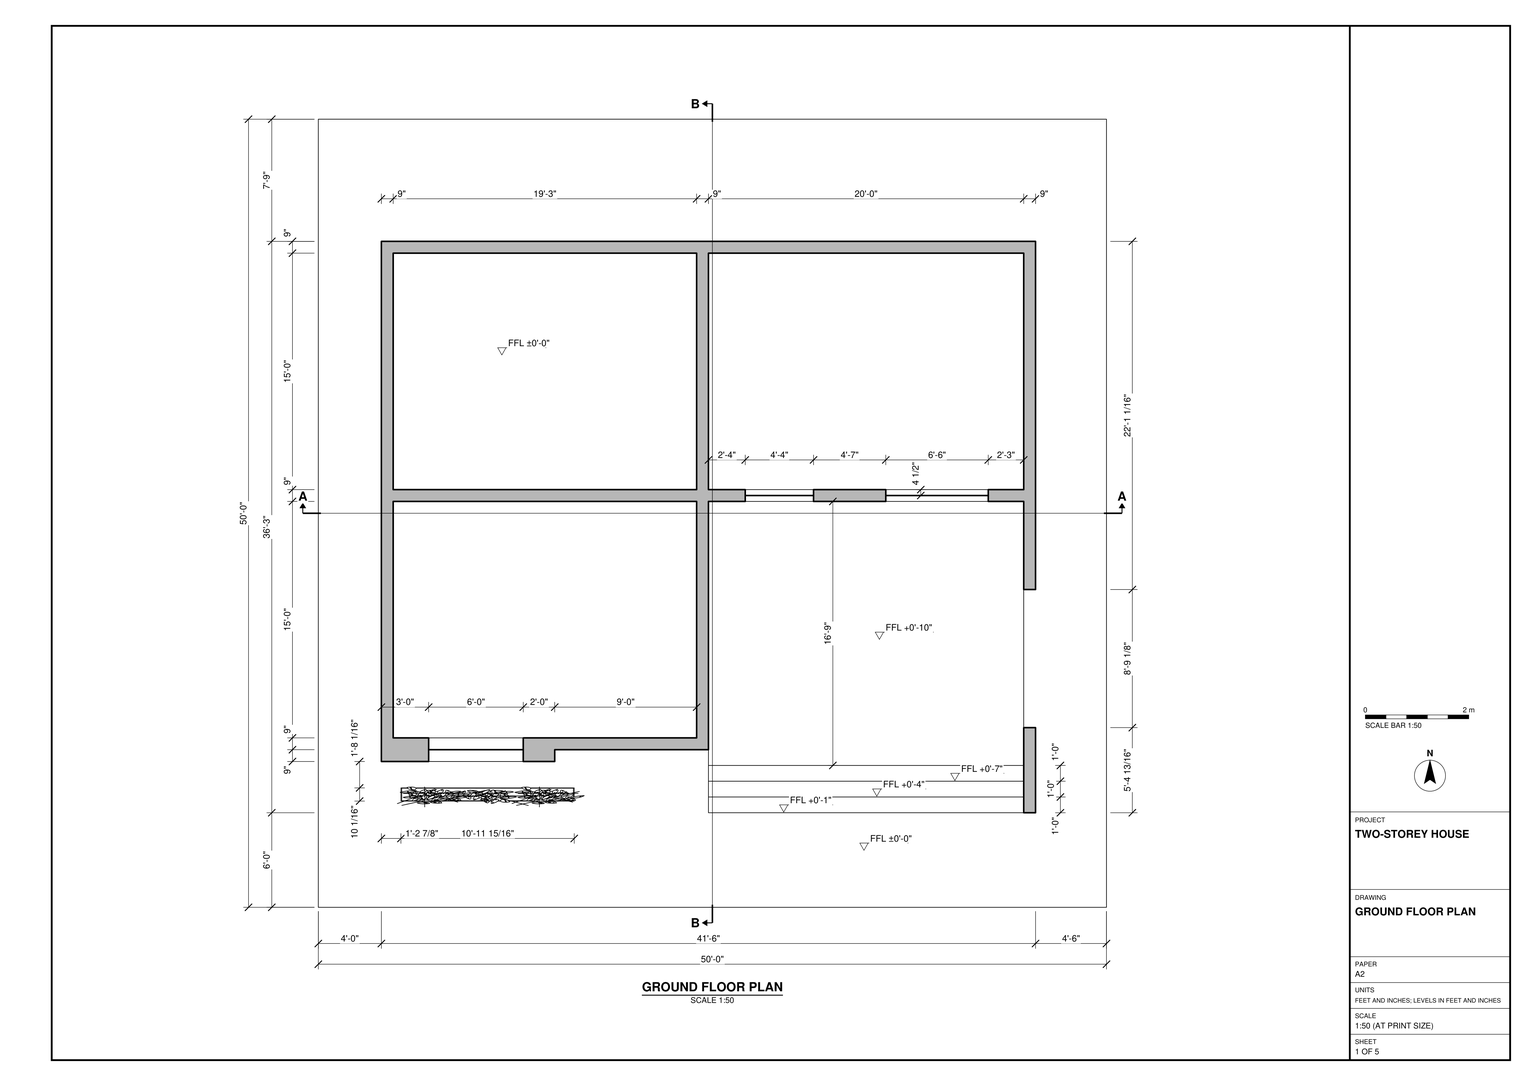
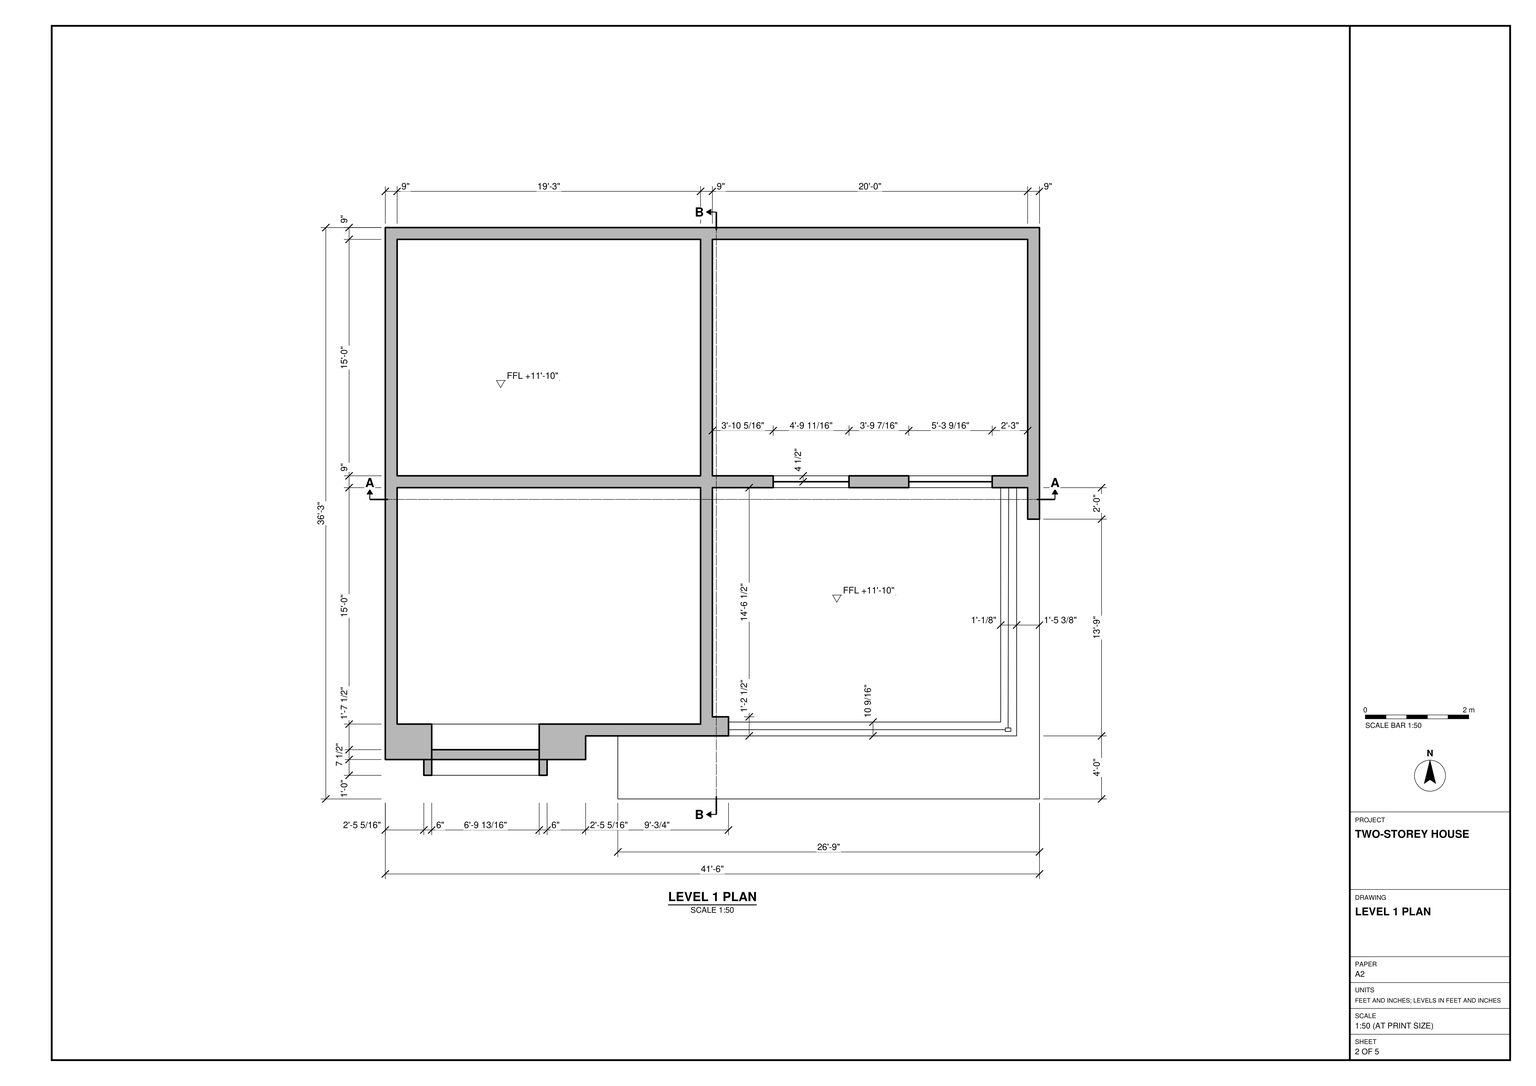
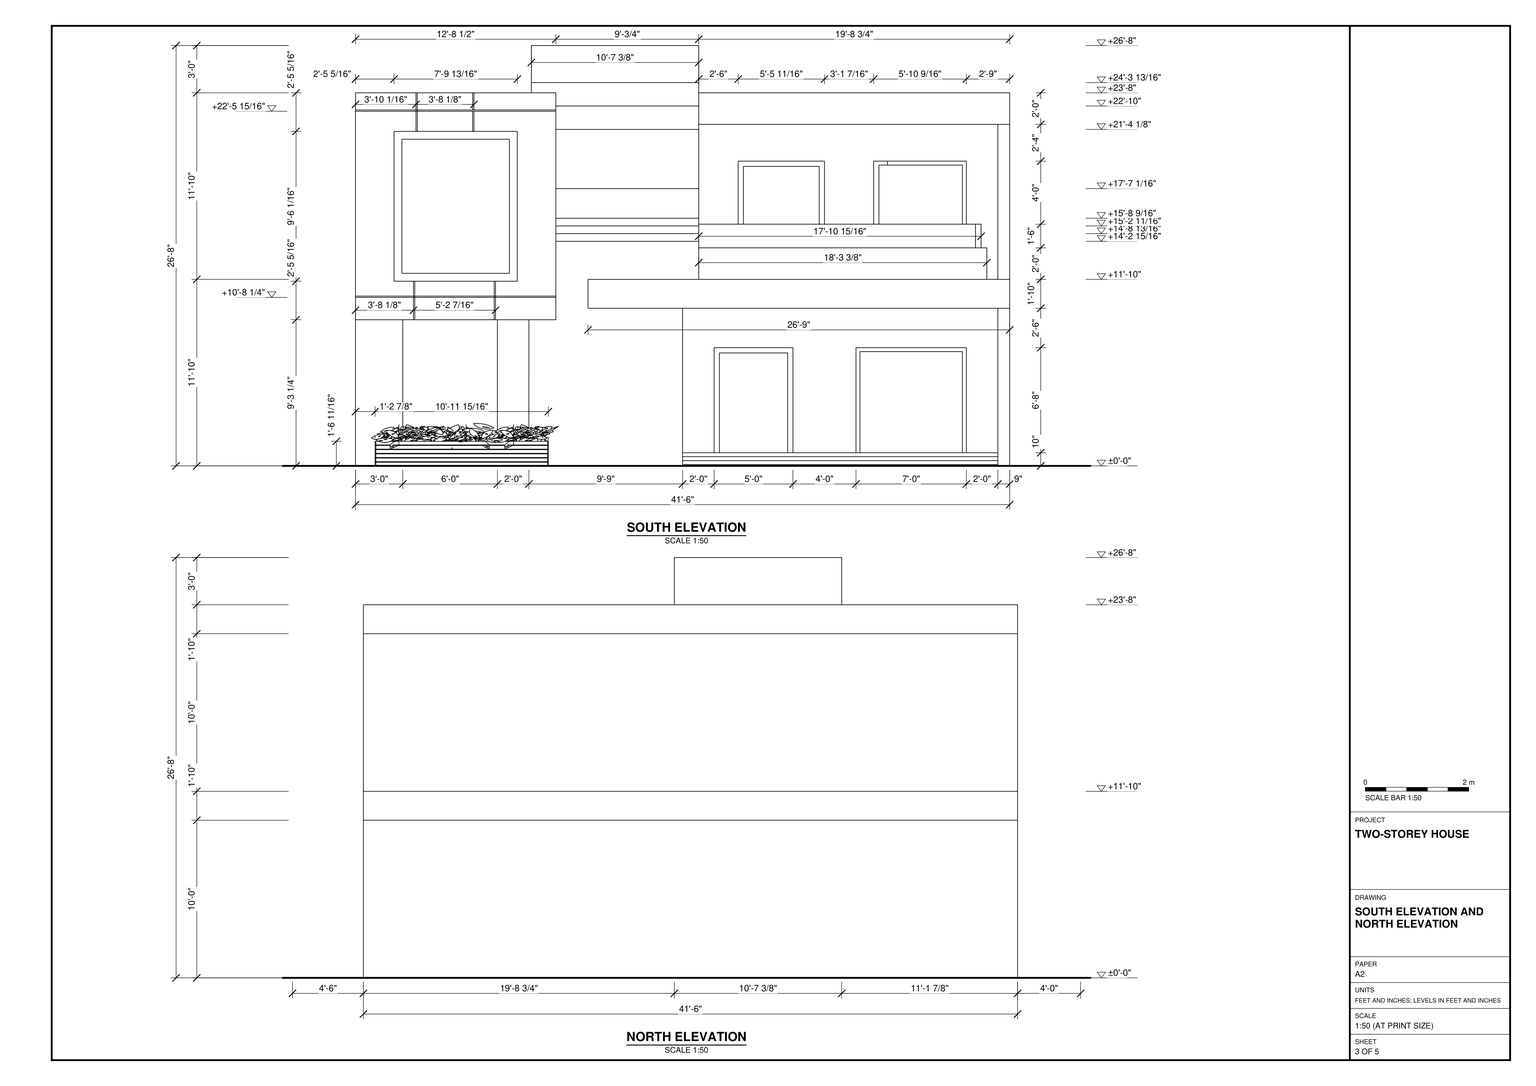
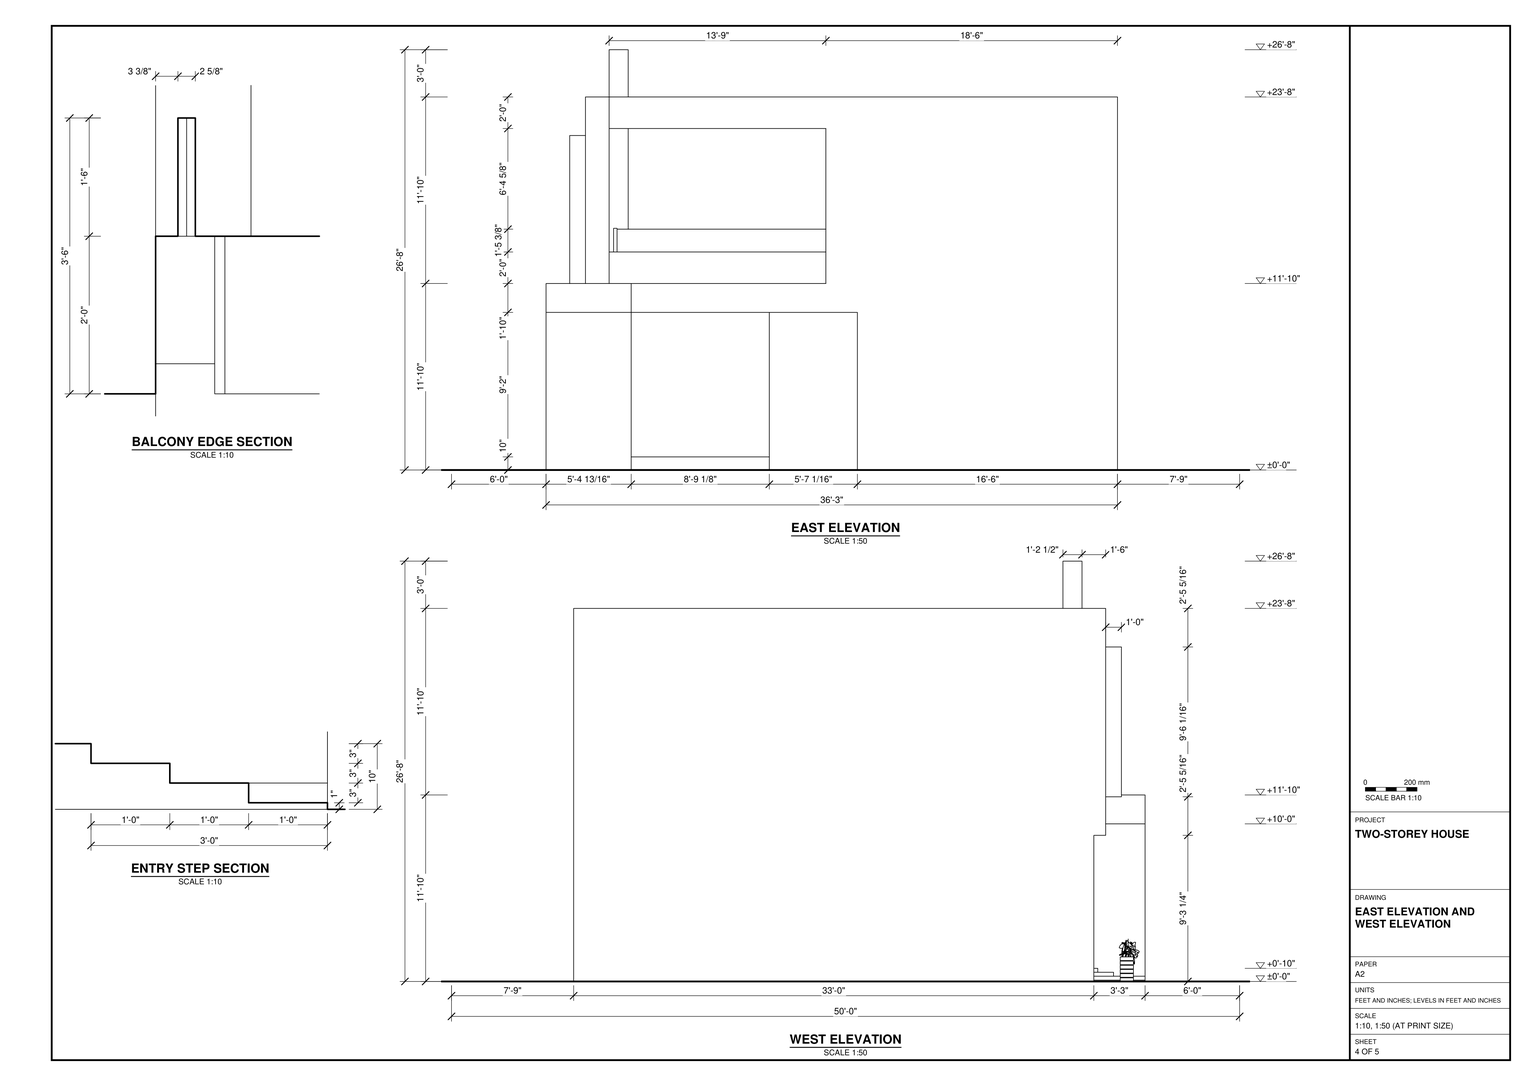
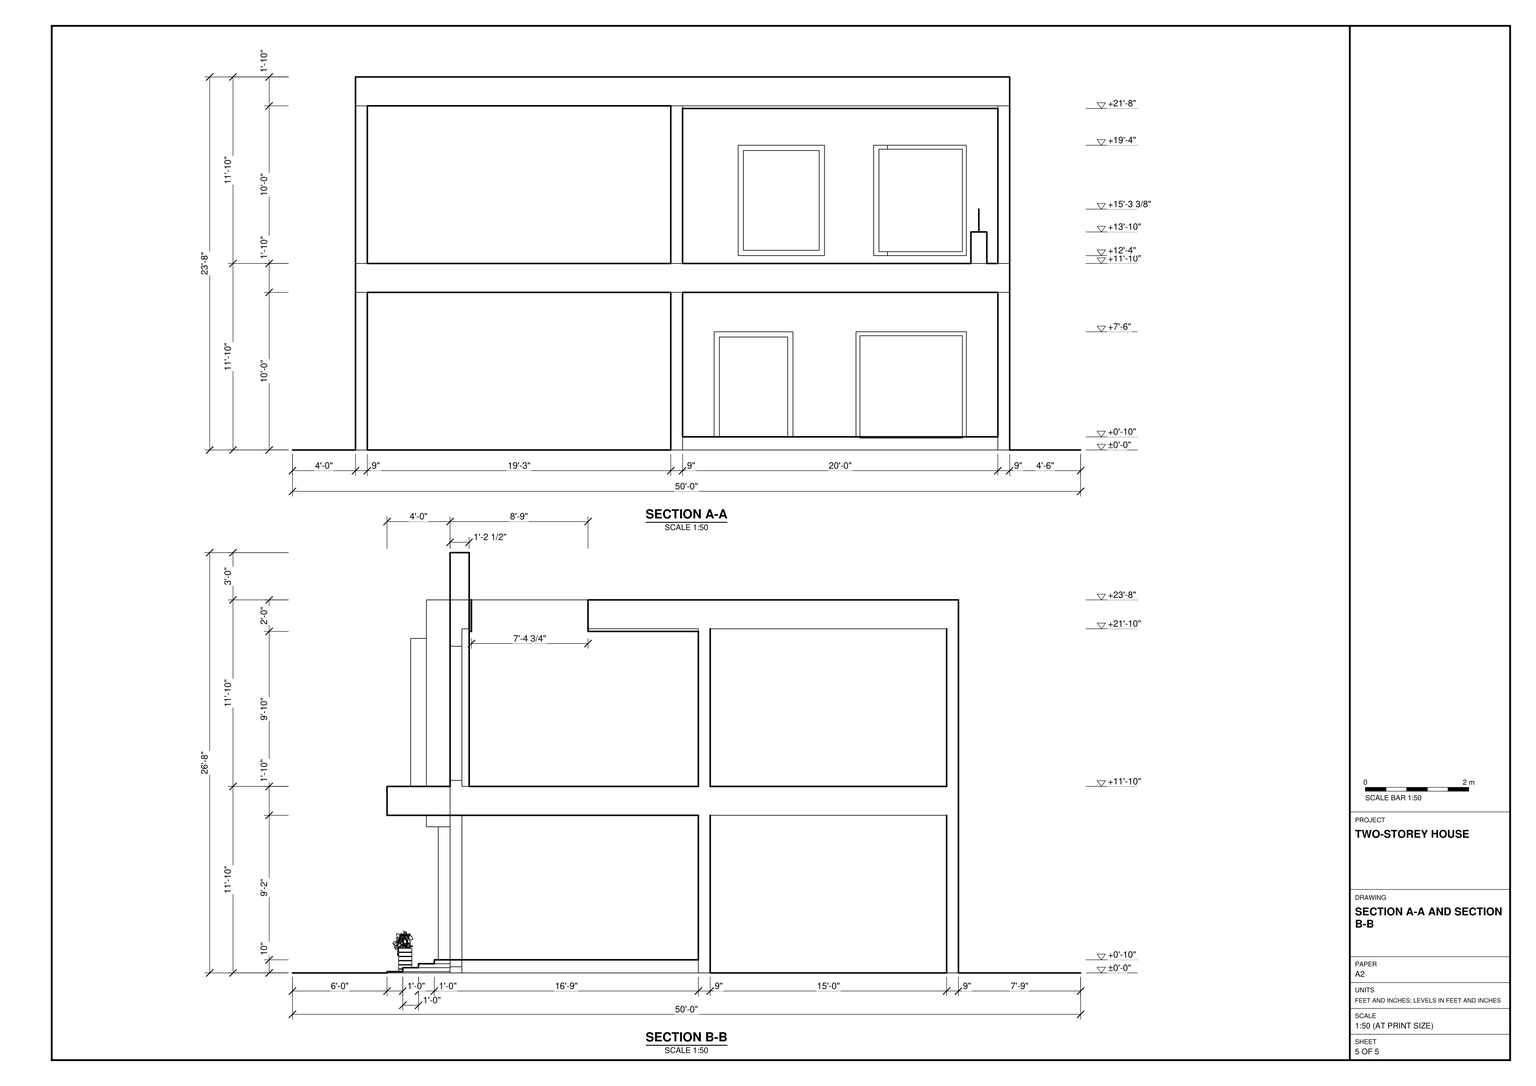
Build the house and its square site in SketchUp from task_files/diagram_01.pdf. Work in feet and inches. The overall model, including the site, is 50'-0" wide by 50'-0" deep by 26'-8" high. Set the ground floor at ±0'-0" and the upper floor at +11'-10". The house is 41'-6" wide, with its west wall 4'-0" from the west site edge and its east wall 4'-6" from the east edge.

Follow the plans for the 9" walls, room divisions and floor slabs. On the south side, form the steps up to the recessed porch and model the balcony directly above it. Place the paired openings in the walls behind the porch and balcony. Match the south elevation for the balcony edge, projecting slab band and deep rectangular frame on the left side of the upper floor. Keep the north wall uninterrupted by openings. Model the flat roof with its raised central portion, and place the planted strip in front of the left bay.

Keep walls, slabs, roof elements and any individual joinery or furniture pieces in separate groups or components. Use components for repeated parts. Planting and other decor or loose items shown may be represented by suitable library components. Save one SketchUp model as output_files/two_storey_house_with_a_recessed_porch_and_balcony.skp.

# SketchUp Ruby script. Lengths in inches.
U = 1.inch
M = Sketchup.active_model
def pt(a) = Geom::Point3d.new(a.map { |v| v * U })
def face(e, loops, mat)
  f = e.add_face(loops[0].map { |a| pt(a) })
  loops[1..].each { |l| e.add_face(l.map { |a| pt(a) }).erase! }
  f.material = f.back_material = mat if mat
  f
end
# faces: each face lists its corners as indices into pts; further lists are holes
def faces(e, pts, list, mat = nil) = list.each { |f| face(e, (f[0].is_a?(Array) ? f : [f]).map { |l| l.map { |i| pts[i] } }, mat) }
# xy, xz, yz: faces in a plane at the given z, y or x. An outline is a flat list of corners, or four numbers for a rectangle; further outlines are holes
def ring(l) = l.size == 4 ? [[l[0], l[1]], [l[2], l[1]], [l[2], l[3]], [l[0], l[3]]] : l.each_slice(2).to_a
def flat(e, list, mat, &to3) = list.each { |f| face(e, (f[0].is_a?(Array) ? f : [f]).map { |l| ring(l).map { |u, v| to3.(u, v) } }, mat) }
def xy(e, z, list, mat = nil) = flat(e, list, mat) { |x, y| [x, y, z] }
def xz(e, y, list, mat = nil) = flat(e, list, mat) { |x, z| [x, y, z] }
def yz(e, x, list, mat = nil) = flat(e, list, mat) { |y, z| [x, y, z] }
def lines(e, pts, list) = list.each { |a, b| e.add_line(pt(pts[a]), pt(pts[b])) }
# prism: a flat outline (further loops are holes) pulled along v
def prism(e, loops, v, mat = nil)
  f = face(e, loops, mat); d = Geom::Vector3d.new(v.map { |x| x * U })
  f.pushpull(f.normal.samedirection?(d) ? d.length : -d.length)
end
def box(e, o, s, mat = nil) = prism(e, [[o, [o[0] + s[0], o[1], o[2]], [o[0] + s[0], o[1] + s[1], o[2]], [o[0], o[1] + s[1], o[2]]]], [0, 0, s[2]], mat)
def at(x, y, z, deg = 0) = Geom::Transformation.translation(pt([x, y, z])) * Geom::Transformation.rotation(ORIGIN, Z_AXIS, deg.degrees)
def axes(o, x, y, z) = Geom::Transformation.new([*x, 0, *y, 0, *z, 0, *pt(o).to_a, 1])
def part(name) = M.definitions.add(name)
# library, detail: a bought-in or finely detailed component or shape, given as its bounding box
def library(name, o, s) = part(name).tap { |d| box(d.entities, o, s) }
def detail(e, o, s) = box(e.add_group.entities, o, s)
def put(e, d, t, mat = nil) = e.add_instance(d, t).tap { |i| i.material = mat if mat }
def group(e, t, mat = nil) = e.add_group.tap { |g| g.transformation = t; g.material = mat if mat }.entities
root = M.entities
M.materials.add("Glass_Basic_01").color = [161, 173, 186]
M.materials["Glass_Basic_01"].alpha = 0.25
M.materials.add("Glass_Mirror_01").color = [185, 116, 75]
M.materials["Glass_Mirror_01"].alpha = 0.6
M.materials.add("M02_Ash_Whisper").color = [185, 196, 188]
M.materials.add("M03_Pewter_Shine").color = [168, 168, 168]
M.materials.add("M06_Steel_Smoke").color = [86, 86, 86]
M.materials.add("Plywood_01_1K").color = [125, 96, 64]
M.materials.add("Wood_Planks_01_1K").color = [69, 67, 63]
M.materials.add("Wood_Veneer_15_1K").color = [103, 69, 45]
c1 = library("Planted timber trough",[0,0,0],[56.02,15.3,25.28])
xy(root,0,[[57,129,288,309],[57,318,288,498],[297,318,537,498]])
xy(root,0,[[[0,0,600,600],[297,72,297,120,179.96,120,179.96,111,48,111,48,507,546,507,546,241.9375,537,241.9375,537,136.8,546,136.8,546,72]]],"M02_Ash_Whisper")
xy(root,1,[[297,72,537,84]])
xy(root,4,[[297,84,537,96]])
xy(root,4.69,[[84,111,156,120],[84,120,156,129]])
xy(root,7,[[297,96,537,108]])
xy(root,9,[[432,309,510,313.5],[432,313.5,510,318]])
xy(root,10,[[297,108,537,309],[325,309,377,313.5],[325,313.5,377,318]])
xy(root,86,[[325,309,377,313.5],[325,313.5,377,318]])
xy(root,87,[[432,309,510,313.5],[432,313.5,510,318]])
xy(root,111.25,[[48,102,48,111,84,111,84,120,156,120,156,111,180,111,180,120,200.49,120,200.49,102],[84,120,156,129]])
xy(root,120,[[225,72,225,120,297,120,297,309,537,309,537,72],[57,129,288,309],[537,136.8,546,241.9375]])
xy(root,140.58,[[77.33,90,171.16,102]])
xy(root,142,[[225,72,546,72,546,285,537,285,537,309,528.61,309,528.61,120,225,120],[57,129,288,309],[309.27,130.55,516.49,130.55,516.49,309,297,309,297,134.52,309.27,134.52],[57,318,288,498],[297,318,537,498]])
xy(root,146.58,[[83.33,90,165.16,109.5],[83.33,109.5,165.16,129]])
xy(root,151,[[446.46,309,510,313.5],[446.46,313.5,510,318]],"Wood_Planks_01_1K")
xy(root,152,[[343.29,313.5,401,318]])
xy(root,152,[[343.29,309,401,313.5]],"Wood_Planks_01_1K")
xy(root,166,[[309.27,120,528.61,120,528.61,309,522.55,309,522.1,126.05,524.22,126.05,524.22,123.4,519.98,123.4,519.98,124.72,309.27,124.72],[309.27,124.72,519.98,124.72,519.98,126.05,522.1,126.05,522.55,309,516.49,309,516.49,130.55,309.27,130.55]])
xy(root,184,[[519.98,123.4,524.22,126.05]])
xy(root,228,[[343.29,309,401,313.5],[343.29,313.5,401,318]],"Wood_Planks_01_1K")
xy(root,229,[[446.46,309,510,313.5],[446.46,313.5,510,318]],"Wood_Planks_01_1K")
xy(root,248.67,[[83.33,90,165.16,109.5],[83.33,109.5,165.16,129]])
xy(root,254.67,[[77.33,90,171.16,102]])
xy(root,260,[[309.27,120,309.27,134.52,297,134.52,297,136.27,537,136.27,537,225,297,225,297,309,537,309,537,285,546,285,546,120]])
xy(root,262,[[57,129,288,309]])
xy(root,284,[[48,102,200.49,120],[48,120,181.87,120,181.87,134.52,297,134.52,297,225,537,225,537,309,546,309,546,507,48,507],[309.27,120,546,120,546,309,537,309,537,136.27,297,136.27,297,134.52,309.27,134.52]])
xy(root,320,[[181.87,120,309.27,134.52]])
xz(root,72,[[297,0,537,1]])
xz(root,72,[[537,0,546,120],[225,120,546,142]],"M06_Steel_Smoke")
xz(root,84,[[297,1,537,4]])
xz(root,90,[[[77.33,140.58,171.16,254.67],[83.33,146.58,165.16,248.67]]])
xz(root,96,[[297,4,537,7]])
xz(root,102,[[92.12,111.25,93.12,128.23],[153.58,111.25,154.58,128.23],[48,128.23,92.12,129.23],[92.12,128.23,93.12,129.23],[93.12,128.23,153.58,129.23],
  [153.58,128.23,154.58,129.23],[154.58,128.23,200.49,129.23],[92.12,129.23,93.12,140.58],[153.58,129.23,154.58,140.58],[94.03,254.67,95.03,269.96],
  [137.16,254.67,138.16,269.96],[48,269.96,94.03,270.96],[94.03,269.96,95.03,270.96],[95.03,269.96,200.49,270.96],[94.03,270.96,95.03,284],
  [137.16,270.96,138.16,284]])
xz(root,102,[[77.33,140.58,171.16,254.67]],"Glass_Mirror_01")
xz(root,102,[[48,111.25,92.12,128.23],[93.12,111.25,153.58,128.23],[154.58,111.25,200.49,128.23],[48,129.23,92.12,129.23,92.12,140.58,77.33,140.58,77.33,254.67,94.03,254.67,94.03,269.96,48,269.96],[93.12,129.23,153.58,140.58],
  [154.58,129.23,200.49,129.23,200.49,269.96,138.16,269.96,138.16,254.67,171.16,254.67,171.16,140.58,154.58,140.58],[95.03,254.67,137.16,269.96],[48,270.96,94.03,284],[95.03,270.96,137.16,284],[138.16,270.96,200.49,284]],"M03_Pewter_Shine")
xz(root,108,[[297,7,537,10]])
xz(root,109.5,[[83.33,146.58,165.16,248.67]],"Glass_Mirror_01")
xz(root,111,[[48,0,156,0,156,4.69,84,4.69,84,111.25,48,111.25]],"M03_Pewter_Shine")
xz(root,111,[[156,0,179.96,0,180,111.25,156,111.25]],"Plywood_01_1K")
xz(root,120,[[84,4.69,156,111.25]],"Glass_Mirror_01")
xz(root,120,[[179.96,0,297,0,297,120,225,120,225,142,309.27,142,309.27,170.96,200.49,170.96,200.49,111.25,180,111.25],[200.49,170.96,309.27,176.82],[200.49,176.82,309.27,182.68],[200.49,182.68,309.27,188.54],[200.49,188.54,309.27,211.08],
  [200.49,211.08,309.27,256.15],[200.49,256.15,309.27,273.98],[200.49,273.98,309.27,273.98,309.27,291.82,181.87,291.82,181.87,284,200.49,284],[181.87,291.82,309.27,320]],"M02_Ash_Whisper")
xz(root,120,[[309.27,142,528.61,166],[309.27,260,546,284]],"M03_Pewter_Shine")
xz(root,123.4,[[519.98,166,524.22,184]])
xz(root,124.72,[[309.27,166,519.98,184]],"Glass_Basic_01")
xz(root,126.05,[[519.98,166,524.22,184]])
xz(root,129,[[[57,0,288,120],[84,4.69,156,111.25]],[[57,142,288,262],[83.33,146.58,165.16,248.67]]])
xz(root,130.55,[[309.27,142,516.49,166]])
xz(root,134.52,[[297,142,309.27,260],[297,260,309.27,284],[181.87,284,309.27,320]])
xz(root,136.27,[[297,260,537,284]])
xz(root,136.8,[[537,0,546,120]])
xz(root,225,[[297,260,537,284]],"M03_Pewter_Shine")
xz(root,241.9375,[[537,0,546,120]],"M03_Pewter_Shine")
xz(root,285,[[537,142,546,260]])
xz(root,309,[[57,0,288,120],[432,9,510,10],[57,142,288,262]])
xz(root,309,[[297,10,321,10,321,90,381,90,381,10,429,10,429,90,513,90,513,10,537,10,537,120,297,120],[[297,142,516.49,142,516.49,166,528.61,166,528.61,142,537,142,537,260,297,260],[442.46,148,513,232],[339.29,148,405,232]]],"M02_Ash_Whisper")
xz(root,309,[[321,10,325,10,325,86,377,86,377,10,381,10,381,90,321,90],[429,10,432,10,432,87,510,87,510,10,513,10,513,90,429,90],[[339.29,148,405,232],[343.29,152,401,228]],[442.46,148,453,148,453,151,446.46,151,446.46,229,453,229,453,232,442.46,232],[453,148,513,148,513,232,453,232,453,229,510,229,510,151,453,151]],"Wood_Planks_01_1K")
xz(root,313.5,[[432,9,510,87],[446.46,151,510,229]],"Glass_Mirror_01")
xz(root,313.5,[[325,10,377,86],[343.29,152,401,228]],"Wood_Veneer_15_1K")
xz(root,318,[[57,0,288,120],[[297,0,537,120],[432,9,510,87],[325,10,377,86]],[57,142,288,262],[[297,142,537,262],[446.46,151,510,229],[343.29,152,401,228]]])
xz(root,498,[[57,0,288,120],[297,0,537,120],[57,142,288,262],[297,142,537,262]])
xz(root,507,[[48,0,546,120],[48,120,546,142],[48,142,546,262],[48,262,546,284]])
yz(root,48,[[111,0,111,111.25,102,111.25,102,284,507,284,507,0]],"M02_Ash_Whisper")
yz(root,57,[[129,0,309,120],[318,0,498,120],[129,142,309,262],[318,142,498,262]])
yz(root,77.33,[[90,140.58,102,254.67]])
yz(root,83.33,[[90,146.58,109.5,248.67],[109.5,146.58,129,248.67]])
yz(root,84,[[111,4.69,120,111.25],[120,4.69,129,111.25]])
yz(root,156,[[120,4.69,129,111.25]])
yz(root,156,[[111,4.69,120,111.25]],"Plywood_01_1K")
yz(root,165.16,[[90,146.58,109.5,248.67],[109.5,146.58,129,248.67]])
yz(root,171.16,[[90,140.58,102,254.67]])
yz(root,181.87,[[120,284,134.52,320]])
yz(root,200.49,[[102,111.25,120,284]])
yz(root,225,[[72,120,120,142]],"M06_Steel_Smoke")
yz(root,288,[[129,0,309,120],[318,0,498,120],[129,142,309,262],[318,142,498,262]])
yz(root,297,[[72,0,120,1],[318,0,498,120],[84,1,120,4],[96,4,120,7],[108,7,120,10],
  [120,10,129,120],[318,142,498,262]])
yz(root,297,[[129,10,309,120],[134.52,142,309,142,309,260,225,260,225,284,136.27,284,136.27,260,134.52,260]],"M02_Ash_Whisper")
yz(root,309.27,[[130.55,142,134.52,142,134.52,260,120,260,120,166,130.55,166],[120,260,134.52,284],[120,284,134.52,320]])
yz(root,325,[[309,10,313.5,86],[313.5,10,318,86]])
yz(root,343.29,[[313.5,152,318,228]])
yz(root,343.29,[[309,152,313.5,228]],"Wood_Planks_01_1K")
yz(root,377,[[309,10,313.5,86],[313.5,10,318,86]])
yz(root,401,[[313.5,152,318,228]])
yz(root,401,[[309,152,313.5,228]],"Wood_Planks_01_1K")
yz(root,432,[[309,9,313.5,87],[313.5,9,318,87]])
yz(root,446.46,[[309,151,313.5,229],[313.5,151,318,229]],"Wood_Planks_01_1K")
yz(root,510,[[309,9,313.5,87],[313.5,9,318,87]])
yz(root,510,[[309,151,313.5,229],[313.5,151,318,229]],"Wood_Planks_01_1K")
yz(root,516.49,[[130.55,142,309,166]])
yz(root,519.98,[[123.4,166,124.72,184],[124.72,166,126.05,184]])
yz(root,524.22,[[123.4,166,126.05,184]])
yz(root,528.61,[[120,142,309,166]],"M03_Pewter_Shine")
yz(root,537,[[136.8,0,241.9375,10],[318,0,498,120],[72,1,84,4],[285,142,309,260],[318,142,498,262],
  [136.27,260,225,284]])
yz(root,537,[[241.9375,10,309,120]],"M03_Pewter_Shine")
yz(root,537,[[72,4,72,120,129,120,129,10,108,10,108,7,96,7,96,4],[129,10,136.8,120]],"M06_Steel_Smoke")
yz(root,546,[[309,0,507,0,507,284,120,284,120,260,285,260,285,142,136.8,142,136.8,120,309,120],[241.9375,0,309,120]],"M03_Pewter_Shine")
yz(root,546,[[72,0,136.8,120],[72,120,136.8,142]],"M06_Steel_Smoke")
p = [[179.96,120,0],[180,120,111.25],[180,111,111.25],[179.96,111,0],[522.1,126.05,166],[522.55,309,166],
  [522.55,309,183.36],[522.1,126.05,183.36],[57,309,262],[48,309,262],[57,309,120],[48,309,120],
  [297,129,120],[288,129,120],[297,129,262],[288,129,262],[181.87,120,273.98],[200.49,120,273.98],
  [181.87,120,256.15],[200.49,120,256.15]]
faces(root,p,[[0,1,2,3]])
faces(root,p,[[4,5,6,7]],"Glass_Basic_01")
lines(root,p,[[8,9],[10,11],[12,13],[14,15],[16,17],[18,19]])
put(root,c1,axes([60.15,76.39,0],[2.54,0,0],[0,1,0],[0,0,1.28]))
